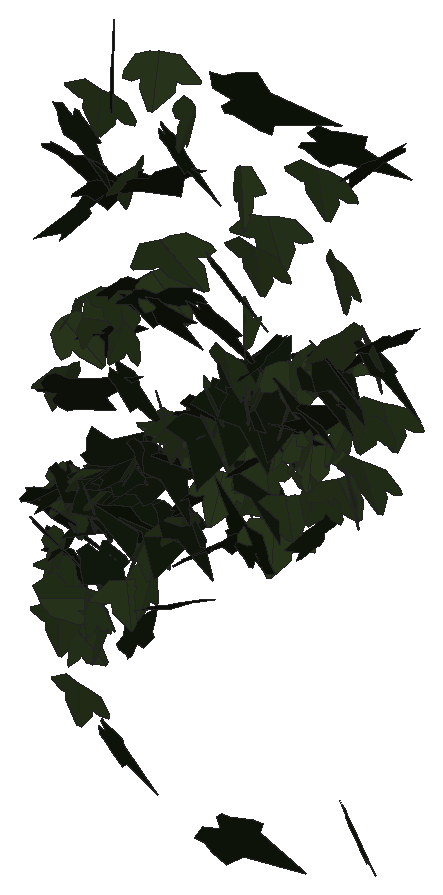
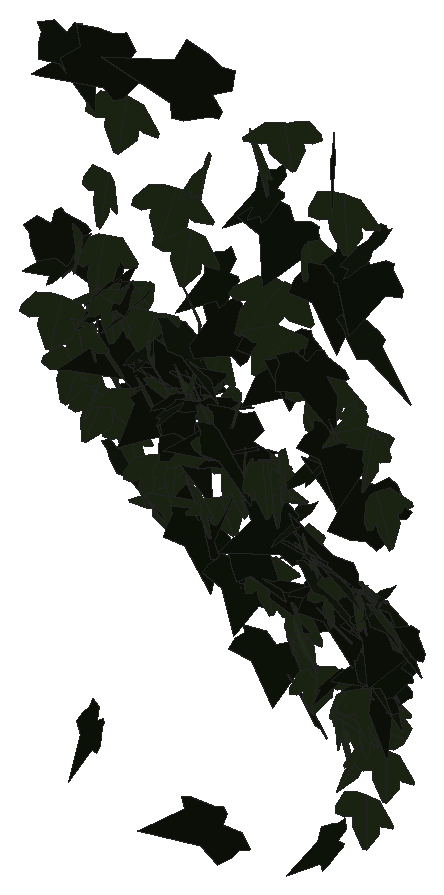
# SketchUp Ruby script. Lengths in inches.
U = 1.inch
M = Sketchup.active_model
def pt(a) = Geom::Point3d.new(a.map { |v| v * U })
def face(e, loops, mat)
  f = e.add_face(loops[0].map { |a| pt(a) })
  loops[1..].each { |l| e.add_face(l.map { |a| pt(a) }).erase! }
  f.material = f.back_material = mat if mat
  f
end
# faces: each face lists its corners as indices into pts; further lists are holes
def faces(e, pts, list, mat = nil) = list.each { |f| face(e, (f[0].is_a?(Array) ? f : [f]).map { |l| l.map { |i| pts[i] } }, mat) }
# xy, xz, yz: faces in a plane at the given z, y or x. An outline is a flat list of corners, or four numbers for a rectangle; further outlines are holes
def ring(l) = l.size == 4 ? [[l[0], l[1]], [l[2], l[1]], [l[2], l[3]], [l[0], l[3]]] : l.each_slice(2).to_a
def flat(e, list, mat, &to3) = list.each { |f| face(e, (f[0].is_a?(Array) ? f : [f]).map { |l| ring(l).map { |u, v| to3.(u, v) } }, mat) }
def xy(e, z, list, mat = nil) = flat(e, list, mat) { |x, y| [x, y, z] }
def xz(e, y, list, mat = nil) = flat(e, list, mat) { |x, z| [x, y, z] }
def yz(e, x, list, mat = nil) = flat(e, list, mat) { |y, z| [x, y, z] }
def lines(e, pts, list) = list.each { |a, b| e.add_line(pt(pts[a]), pt(pts[b])) }
# prism: a flat outline (further loops are holes) pulled along v
def prism(e, loops, v, mat = nil)
  f = face(e, loops, mat); d = Geom::Vector3d.new(v.map { |x| x * U })
  f.pushpull(f.normal.samedirection?(d) ? d.length : -d.length)
end
def box(e, o, s, mat = nil) = prism(e, [[o, [o[0] + s[0], o[1], o[2]], [o[0] + s[0], o[1] + s[1], o[2]], [o[0], o[1] + s[1], o[2]]]], [0, 0, s[2]], mat)
def at(x, y, z, deg = 0) = Geom::Transformation.translation(pt([x, y, z])) * Geom::Transformation.rotation(ORIGIN, Z_AXIS, deg.degrees)
def axes(o, x, y, z) = Geom::Transformation.new([*x, 0, *y, 0, *z, 0, *pt(o).to_a, 1])
def part(name) = M.definitions.add(name)
# library, detail: a bought-in or finely detailed component or shape, given as its bounding box
def library(name, o, s) = part(name).tap { |d| box(d.entities, o, s) }
def detail(e, o, s) = box(e.add_group.entities, o, s)
def put(e, d, t, mat = nil) = e.add_instance(d, t).tap { |i| i.material = mat if mat }
def group(e, t, mat = nil) = e.add_group.tap { |g| g.transformation = t; g.material = mat if mat }.entities
root = M.entities
M.materials.add("1026 AP 7946 SUNNY SIDE UP").color = [254, 231, 186]
M.materials.add("efeu1").color = [18, 25, 13]
M.materials.add("efeu2").color = [43, 57, 29]
c1 = part("ivyleaf_9")
p = [[1.54,2.16,1.25],[1.36,2.04,1.19],[-0.21,0.99,0.68],[-0.71,1.11,0.82],[-0.85,0.86,0.67],[-0.8,0.17,0.21],
  [-0.9,-0.01,0.1],[-0.67,-0.16,-0.02],[-0.08,-0.08,-0.05],[-0.03,-0.6,-0.4],[0.65,-0.88,-0.66],[0.83,-0.6,-0.49],
  [1.29,-0.42,-0.43],[1.8125,-0.07,-0.26],[1.21,0.44,0.15]]
faces(c1.entities,p,[[0,1,2,3,4,5,6,7,8,9,10,11,12,13,14]],"efeu1")
c2 = part("ivyleaf_10")
p = [[0,0.5,-0.03],[-0.0625,2.02,-0.43],[-0.19,2.01,-0.46],[-0.54,1.05,-0.29],[-0.52,0.625,-0.18],[-0.83,0.76,-0.28],
  [-1.16,0.64,-0.33],[-1.15,0.33,-0.24],[-0.77,-0.39,0.02],[-0.3,-0.51,0.16],[0.04,-0.48,0.23],[-0.02,2.01,-0.4375],
  [-0.06,2.01,-0.43],[0.04,-0.49,0.23],[0.67,-0.49,0.14],[1.38,0.36,-0.2],[1.375,0.51,-0.24],[0.81,0.65,-0.19],
  [0.62,0.59,-0.15],[0.6,1.09,-0.28],[0.5,1.23,-0.31]]
faces(c2.entities,p,[[0,1,2,3,4,5,6,7,8,9,10],[11,12,0,13,14,15,16,17,18,19,20]],"efeu2")
put(root,c1,axes([122.53,212.98,271.5625],[0.22662,-0.02057,-0.23911],[-0.36508,0.00859,-0.14934],[0.02856,0.27297,-0.01171]),"1026 AP 7946 SUNNY SIDE UP")
put(root,c2,axes([122.51,212.89,270.52],[-0.4181,0.04854,0.03929],[-0.06821,-0.02864,-0.27619],[-0.06868,-0.26705,0.03513]),"1026 AP 7946 SUNNY SIDE UP")
put(root,c1,axes([122.42,212.8125,272.46],[0.27398,0.21836,-0.00939],[0.003,-0.01477,-0.28767],[-0.34373,0.17392,-0.01]),"1026 AP 7946 SUNNY SIDE UP")
put(root,c1,axes([122.69,212.7,272.61],[-0.18146,0.2621,0.02234],[-0.03851,0.01125,-0.29439],[-0.41154,-0.11662,0.01769]),"1026 AP 7946 SUNNY SIDE UP")
put(root,c2,axes([122.48,212.86,271.68],[0.2605,-0.21806,0.00555],[0.00539,-0.00571,-0.28216],[0.343,0.1657,0.00022]),"1026 AP 7946 SUNNY SIDE UP")
put(root,c1,axes([122.22,212.87,271.77],[0.34565,-0.16054,0.06421],[0.08155,-0.03622,-0.28063],[0.25877,0.22585,0.00267]),"1026 AP 7946 SUNNY SIDE UP")
put(root,c1,axes([122.22,212.97,272.04],[0.39548,-0.09969,0.06037],[0.0993,-0.0007,-0.27779],[0.15286,0.25838,0.02427]),"1026 AP 7946 SUNNY SIDE UP")
put(root,c1,axes([122.72,212.87,271.83],[-0.14965,0.25687,0.02102],[-0.01059,0.01771,-0.2821],[-0.40485,-0.09541,-0.00039]),"1026 AP 7946 SUNNY SIDE UP")
put(root,c2,axes([122.61,212.83,274.26],[-0.0857,-0.28398,0.0248],[0.00631,-0.02691,-0.29791],[0.44831,-0.05391,0.00894]),"1026 AP 7946 SUNNY SIDE UP")
put(root,c2,axes([122.68,212.96,271.38],[-0.35392,-0.15518,0.00923],[0.01173,-0.02808,-0.2804],[0.24422,-0.22354,0.02685]),"1026 AP 7946 SUNNY SIDE UP")
put(root,c2,axes([122.67,212.89,272.67],[0.34306,-0.17608,-0.00482],[-0.02989,-0.01772,-0.28772],[0.27531,0.21749,-0.02523]),"1026 AP 7946 SUNNY SIDE UP")
put(root,c1,axes([122.95,212.88,276.79],[-0.28904,0.26922,-0.05345],[0.02471,-0.05386,-0.33568],[-0.43086,-0.18369,0.01661]),"1026 AP 7946 SUNNY SIDE UP")
put(root,c2,axes([122.73,212.84,272.46],[-0.43019,0.06143,-0.01948],[0.01444,-0.04598,-0.28576],[-0.10019,-0.27038,0.04246]),"1026 AP 7946 SUNNY SIDE UP")
put(root,c2,axes([122.72,212.84,275.11],[0.01575,-0.25454,-0.15111],[0.06267,0.14515,-0.2584],[0.45653,-0.01114,0.04069]),"1026 AP 7946 SUNNY SIDE UP")
put(root,c2,axes([122.49,212.77,270.88],[-0.12444,-0.04589,0.27298],[0.31916,0.17142,0.09395],[-0.27802,0.21733,-0.01434]),"1026 AP 7946 SUNNY SIDE UP")
put(root,c2,axes([122.84,212.89,272.71],[0.02726,-0.28212,0.00318],[-0.00747,-0.00499,-0.29117],[0.4436,0.01725,-0.0051]),"1026 AP 7946 SUNNY SIDE UP")
put(root,c2,axes([122.93,212.78,269.65],[-0.41498,0.05647,0.05341],[-0.08683,-0.01276,-0.27705],[-0.08312,-0.2686,0.02274]),"1026 AP 7946 SUNNY SIDE UP")
put(root,c1,axes([122.67,212.86,272.75],[0.22083,-0.23889,-0.06244],[-0.02541,0.05912,-0.28468],[0.38618,0.1405,0.01697]),"1026 AP 7946 SUNNY SIDE UP")
put(root,c1,axes([122.91,212.72,277.63],[0.39161,0.12084,-0.14425],[-0.24313,0.00515,-0.27735],[-0.16108,0.28601,0.06792]),"1026 AP 7946 SUNNY SIDE UP")
put(root,c2,axes([123,212.89,270.93],[-0.37994,0.12302,0.04689],[-0.12258,-0.0596,-0.26481],[-0.1654,-0.23842,0.08853]),"1026 AP 7946 SUNNY SIDE UP")
put(root,c1,axes([122.7,212.93,278.03],[0.19808,-0.2736,0.03914],[0.0193,-0.03788,-0.31049],[0.43425,0.12648,-0.00405]),"1026 AP 7946 SUNNY SIDE UP")
put(root,c1,axes([122.64,212.73,274.01],[0.37365,0.20279,-0.10254],[0.0843,0.09141,0.32056],[0.34589,-0.24135,0.03264]),"1026 AP 7946 SUNNY SIDE UP")
put(root,c2,axes([122.96,212.8,272.7],[-0.23019,0.23958,-0.02362],[-0.00051,-0.02862,-0.28899],[-0.37865,-0.14561,0.01475]),"1026 AP 7946 SUNNY SIDE UP")
put(root,c2,axes([122.86,212.68,275.07],[0.16423,0.22664,0.16237],[0.09304,0.14481,-0.25617],[-0.42281,0.1199,0.0067]),"1026 AP 7946 SUNNY SIDE UP")
put(root,c2,axes([122.93,212.82,270.44],[-0.01642,-0.23407,-0.1501],[0.16525,0.13011,-0.2244],[0.39961,-0.06343,0.08663]),"1026 AP 7946 SUNNY SIDE UP")
put(root,c1,axes([123.12,212.94,272.7],[0.25806,0.17161,-0.15313],[-0.14303,-0.11965,-0.24488],[-0.32818,0.18709,-0.01369]),"1026 AP 7946 SUNNY SIDE UP")
put(root,c2,axes([123.18,212.92,278.52],[-0.471,0.01526,0.05824],[-0.09073,-0.02956,-0.30741],[-0.01485,-0.30338,0.03108]),"1026 AP 7946 SUNNY SIDE UP")
put(root,c1,axes([123.16,212.91,275.02],[0.15872,0.2741,-0.01722],[0.0043,-0.02047,-0.30087],[-0.43193,0.10052,-0.00932]),"1026 AP 7946 SUNNY SIDE UP")
put(root,c2,axes([123.24,212.85,271.09],[-0.22518,0.18129,0.15871],[-0.1698,0.10934,-0.23692],[-0.33215,-0.1788,0.01353]),"1026 AP 7946 SUNNY SIDE UP")
put(root,c1,axes([123.35,213.01,272.41],[-0.38475,0.12561,-0.03026],[0.02544,-0.03414,-0.28257],[-0.2015,-0.24416,0.02211]),"1026 AP 7946 SUNNY SIDE UP")
put(root,c2,axes([123.17,212.95,272.86],[-0.31044,-0.18987,-0.04619],[0.08707,0.00506,-0.27994],[0.29375,-0.20216,0.03416]),"1026 AP 7946 SUNNY SIDE UP")
put(root,c2,axes([123.13,212.69,275.34],[0.0015,-0.14596,-0.26552],[0.15493,0.24236,-0.14006],[0.43801,-0.08523,0.05045]),"1026 AP 7946 SUNNY SIDE UP")
put(root,c2,axes([123.29,212.77,270.61],[0.16619,-0.24356,-0.07999],[-0.0398,0.07213,-0.27304],[0.39933,0.10855,0.00608]),"1026 AP 7946 SUNNY SIDE UP")
put(root,c2,axes([123.27,212.93,272.65],[0.00886,-0.27426,0.05014],[0.02142,-0.04991,-0.2826],[0.43789,0.00799,0.01281]),"1026 AP 7946 SUNNY SIDE UP")
put(root,c1,axes([123.11,212.96,271.67],[0.11195,-0.23955,-0.11981],[-0.05845,0.10884,-0.25678],[0.41367,0.08021,-0.00386]),"1026 AP 7946 SUNNY SIDE UP")
put(root,c1,axes([123.33,212.89,277.34],[0.13376,0.28654,-0.04761],[-0.01271,-0.0475,-0.30815],[-0.45662,0.08526,-0.00537]),"1026 AP 7946 SUNNY SIDE UP")
put(root,c1,axes([123.57,212.96,272.94],[-0.22552,0.2392,0.02733],[-0.04485,0.01219,-0.28665],[-0.37553,-0.1451,0.01782]),"1026 AP 7946 SUNNY SIDE UP")
put(root,c1,axes([123.47,212.74,278.71],[0.01476,-0.09243,0.32751],[0.08567,0.31467,0.09428],[-0.5143,0.04976,0.0251]),"1026 AP 7946 SUNNY SIDE UP")
put(root,c2,axes([123.58,212.88,275.2],[-0.34307,0.17362,0.10312],[-0.21622,-0.02384,-0.26896],[-0.22818,-0.23845,0.09983]),"1026 AP 7946 SUNNY SIDE UP")
put(root,c1,axes([123.72,212.9,273.18],[-0.35005,0.16297,0.04746],[-0.11718,-0.02755,-0.27629],[-0.23869,-0.22548,0.06603]),"1026 AP 7946 SUNNY SIDE UP")
put(root,c1,axes([123.68,212.82,273.24],[-0.18259,0.24752,0.06637],[-0.09761,0.0398,-0.27865],[-0.38958,-0.12598,0.03871]),"1026 AP 7946 SUNNY SIDE UP")
put(root,c1,axes([123.28,212.93,269.0625],[0.32843,-0.17099,-0.07704],[-0.07189,0.06044,-0.27717],[0.28389,0.21313,0.01894]),"1026 AP 7946 SUNNY SIDE UP")
put(root,c1,axes([123.31,212.93,273.03],[-0.2044,0.12307,0.22651],[0.26161,-0.14283,0.18345],[0.29627,0.21103,-0.00571]),"1026 AP 7946 SUNNY SIDE UP")
put(root,c2,axes([123.54,212.87,275.68],[-0.41037,-0.1408,-0.00756],[0.02713,-0.01825,-0.30458],[0.21996,-0.26043,0.02346]),"1026 AP 7946 SUNNY SIDE UP")
put(root,c1,axes([123.39,212.875,272.74],[-0.13371,-0.23152,-0.14557],[0.08717,0.12872,-0.25325],[0.4164,-0.10129,0.00627]),"1026 AP 7946 SUNNY SIDE UP")
put(root,c1,axes([123.73,212.92,275.98],[0.01893,0.26471,-0.1366],[-0.00313,-0.13414,-0.27375],[-0.46659,0.01164,-0.0037]),"1026 AP 7946 SUNNY SIDE UP")
put(root,c2,axes([123.61,212.89,271.37],[-0.23173,-0.2347,-0.00504],[0.11421,-0.04161,-0.27243],[0.35096,-0.14142,0.08533]),"1026 AP 7946 SUNNY SIDE UP")
put(root,c2,axes([123.69,212.89,277.6],[0.00022,-0.30207,-0.03698],[0.02241,0.03415,-0.31065],[0.47748,-0.00147,0.0146]),"1026 AP 7946 SUNNY SIDE UP")
put(root,c1,axes([123.96,212.97,273.1875],[-0.41614,0.06145,0.06559],[-0.11207,-0.03085,-0.27622],[-0.0818,-0.27037,0.04474]),"1026 AP 7946 SUNNY SIDE UP")
put(root,c2,axes([123.73,212.91,273.35],[0.12216,-0.27441,-0.00467],[-0.00148,0.00283,-0.29379],[0.43151,0.0777,0.00032]),"1026 AP 7946 SUNNY SIDE UP")
put(root,c2,axes([123.77,213.04,272.1],[0.13573,-0.26106,0.02199],[-0.00235,-0.02453,-0.28325],[0.41205,0.08586,-0.00886]),"1026 AP 7946 SUNNY SIDE UP")
put(root,c1,axes([123.92,212.71,270.78],[0.02853,0.1117,0.26242],[-0.08119,0.25155,-0.10865],[-0.42882,-0.0402,0.03803]),"1026 AP 7946 SUNNY SIDE UP")
put(root,c1,axes([123.59,212.8,274.57],[0.31078,-0.1877,-0.10864],[-0.08245,0.09541,-0.27843],[0.3275,0.20214,0.033]),"1026 AP 7946 SUNNY SIDE UP")
put(root,c1,axes([123.5,212.8125,272.35],[0.22303,-0.05599,0.23681],[0.34559,-0.06904,-0.15722],[0.13903,0.26142,0.01091]),"1026 AP 7946 SUNNY SIDE UP")
put(root,c2,axes([123.96,212.87,271.65],[0.32907,-0.18368,0.02519],[0.04112,-0.00883,-0.2867],[0.28867,0.21064,0.01212]),"1026 AP 7946 SUNNY SIDE UP")
put(root,c2,axes([123.93,212.9,272.16],[0.3955,-0.11882,0.03464],[0.08854,0.04083,-0.27948],[0.17313,0.25055,0.0638]),"1026 AP 7946 SUNNY SIDE UP")
put(root,c2,axes([124.09,212.94,279.33],[0.33872,0.21842,-0.03574],[-0.06636,-0.00869,-0.31514],[-0.34168,0.21822,0.02578]),"1026 AP 7946 SUNNY SIDE UP")
put(root,c1,axes([123.94,212.9,273.56],[0.24274,-0.23659,-0.04875],[0.00307,0.05583,-0.28887],[0.37897,0.15109,0.03356]),"1026 AP 7946 SUNNY SIDE UP")
put(root,c1,axes([124.01,212.76,275.82],[0.46248,0.04372,-0.00493],[-0.00837,0.00163,-0.30631],[-0.06869,0.29416,0.00418]),"1026 AP 7946 SUNNY SIDE UP")
put(root,c1,axes([124.28,212.69,276.08],[0.19879,0.25686,-0.09471],[-0.06036,-0.08519,-0.29541],[-0.42549,0.13209,-0.00234]),"1026 AP 7946 SUNNY SIDE UP")
put(root,c2,axes([124.31,212.74,274.22],[0.11696,-0.13389,-0.2521],[-0.0805,0.24162,-0.15128],[0.43009,0.08163,0.04024]),"1026 AP 7946 SUNNY SIDE UP")
put(root,c1,axes([124.2,212.67,277.79],[0.24345,0.26572,0.05119],[0.03819,0.04162,-0.31658],[-0.42291,0.15672,0.00088]),"1026 AP 7946 SUNNY SIDE UP")
put(root,c1,axes([124.24,213.01,272.6],[-0.31463,-0.18184,-0.07247],[0.12961,0.01086,-0.27443],[0.27718,-0.21148,0.04607]),"1026 AP 7946 SUNNY SIDE UP")
put(root,c1,axes([124.05,212.91,273.41],[0.35077,0.09967,0.14115],[0.17449,0.084,-0.24962],[-0.20036,0.24764,0.02972]),"1026 AP 7946 SUNNY SIDE UP")
put(root,c1,axes([124.42,212.76,271.48],[0.16466,0.25888,0.01615],[-0.09402,0.03903,-0.27828],[-0.39668,0.09821,0.07266]),"1026 AP 7946 SUNNY SIDE UP")
put(root,c1,axes([124.18,212.98,273.5],[0.0895,-0.27643,-0.00918],[-0.00391,0.00698,-0.29071],[0.4348,0.05697,-0.00073]),"1026 AP 7946 SUNNY SIDE UP")
put(root,c2,axes([124.21,212.83,276.15],[0.23369,0.21091,0.15598],[0.09697,0.13938,-0.26365],[-0.39543,0.15882,0.02752]),"1026 AP 7946 SUNNY SIDE UP")
put(root,c2,axes([124.39,212.87,274.04],[0.31435,-0.18421,-0.10323],[-0.03272,0.11897,-0.2702],[0.32731,0.1888,0.07213]),"1026 AP 7946 SUNNY SIDE UP")
put(root,c2,axes([124.43,212.96,274.15],[-0.16461,-0.26685,-0.02071],[0.02313,0.01419,-0.29509],[0.41998,-0.10537,0.00813]),"1026 AP 7946 SUNNY SIDE UP")
put(root,c2,axes([124.71,212.9,273.98],[0.09063,-0.02861,-0.28955],[-0.43412,0.05435,-0.06374],[0.093,0.28156,-0.01539]),"1026 AP 7946 SUNNY SIDE UP")
put(root,c2,axes([124.48,212.9,272.65],[-0.14711,-0.266,0.00922],[0.00787,-0.01285,-0.29042],[0.41851,-0.09326,0.00871]),"1026 AP 7946 SUNNY SIDE UP")
put(root,c2,axes([124.38,212.8,276.75],[-0.37433,-0.18716,-0.1729],[0.24526,0.06946,-0.30927],[0.30858,-0.28225,0.03607]),"1026 AP 7946 SUNNY SIDE UP")
put(root,c2,axes([124.56,212.88,274.12],[-0.0632,-0.28561,0.02529],[0.00224,-0.02662,-0.29724],[0.45097,-0.03989,0.00502]),"1026 AP 7946 SUNNY SIDE UP")
put(root,c1,axes([124.62,213.1,273.07],[-0.14296,0.19611,-0.18246],[0.10377,-0.16573,-0.22352],[-0.40355,-0.11209,0.00716]),"1026 AP 7946 SUNNY SIDE UP")
put(root,c1,axes([124.34,212.86,278.33],[0.36262,-0.18799,-0.07964],[-0.08484,0.05443,-0.30609],[0.30749,0.23671,0.00946]),"1026 AP 7946 SUNNY SIDE UP")
put(root,c1,axes([124.39,212.96,272.74],[0.14282,-0.25807,-0.06234],[-0.00789,0.06074,-0.28107],[0.41621,0.08971,0.01607]),"1026 AP 7946 SUNNY SIDE UP")
put(root,c2,axes([124.67,212.83,278.82],[0.28075,-0.25454,-0.02477],[0.00565,0.03007,-0.31945],[0.40177,0.17745,0.0218]),"1026 AP 7946 SUNNY SIDE UP")
put(root,c1,axes([124.88,212.85,272.39],[0.10384,0.26336,0.08493],[-0.0028,0.08365,-0.27837],[-0.43322,0.06258,0.02216]),"1026 AP 7946 SUNNY SIDE UP")
put(root,c2,axes([124.89,212.97,274],[-0.07039,-0.28131,0.00393],[0.00132,-0.00561,-0.29348],[0.44242,-0.04474,0.0015]),"1026 AP 7946 SUNNY SIDE UP")
put(root,c1,axes([125.125,212.98,274.46],[-0.10653,0.27541,-0.02646],[-0.00176,-0.02832,-0.29224],[-0.43516,-0.06731,0.00766]),"1026 AP 7946 SUNNY SIDE UP")
put(root,c1,axes([125,212.97,274.19],[-0.20783,-0.25012,0.01763],[0.002,-0.02162,-0.29134],[0.39437,-0.13171,0.01076]),"1026 AP 7946 SUNNY SIDE UP")
put(root,c1,axes([124.77,212.85,274.45],[0.35382,0.06499,0.18281],[0.27268,0.03719,-0.24086],[-0.11671,0.28392,-0.00852]),"1026 AP 7946 SUNNY SIDE UP")
put(root,c2,axes([125.12,212.73,274.85],[-0.25989,0.23751,0.03166],[-0.03534,0.02014,-0.29789],[-0.37465,-0.16666,0.00614]),"1026 AP 7946 SUNNY SIDE UP")
put(root,c2,axes([125.06,212.84,274.29],[-0.34345,0.16434,-0.09913],[0.10394,-0.0734,-0.28143],[-0.28163,-0.22751,0.01703]),"1026 AP 7946 SUNNY SIDE UP")
put(root,c2,axes([125.13,212.95,273.45],[0.28767,0.20395,-0.07156],[-0.07182,-0.05389,-0.28256],[-0.33169,0.18855,-0.00088]),"1026 AP 7946 SUNNY SIDE UP")
put(root,c1,axes([125,212.77,276.02],[0.45615,-0.07835,0.00611],[-0.00189,-0.02882,-0.30837],[0.12358,0.28873,-0.02729]),"1026 AP 7946 SUNNY SIDE UP")
put(root,c2,axes([125.2,212.97,274.31],[-0.00103,-0.28061,0.05616],[-0.00105,0.05611,0.28941],[-0.44996,0.00051,-0.00081]),"1026 AP 7946 SUNNY SIDE UP")
put(root,c2,axes([125.42,212.77,275.4375],[-0.41318,0.14647,0.00058],[-0.02317,-0.02699,-0.30845],[-0.22914,-0.26138,0.03015]),"1026 AP 7946 SUNNY SIDE UP")
put(root,c1,axes([125.2,212.78,276.75],[0.39129,-0.15497,-0.07044],[-0.09079,0.03497,-0.3018],[0.2498,0.25546,0.00065]),"1026 AP 7946 SUNNY SIDE UP")
put(root,c1,axes([125.6,212.85,272.93],[0.03028,0.28375,-0.02797],[0.00023,-0.02884,-0.29315],[-0.44846,0.01915,-0.00204]),"1026 AP 7946 SUNNY SIDE UP")
put(root,c2,axes([125.53,213.04,273.5],[0.28375,-0.21296,-0.04515],[-0.03956,0.03453,-0.28734],[0.3392,0.18218,0.00425]),"1026 AP 7946 SUNNY SIDE UP")
put(root,c1,axes([125.5,212.94,274.8],[-0.254,-0.23795,-0.03618],[0.0545,0.0172,-0.29555],[0.37396,-0.16413,0.0185]),"1026 AP 7946 SUNNY SIDE UP")
put(root,c2,axes([125.55,212.97,274.12],[0.16927,0.24316,-0.1028],[-0.07392,-0.0898,-0.2744],[-0.40747,0.1173,0.00708]),"1026 AP 7946 SUNNY SIDE UP")
put(root,c2,axes([125.72,212.76,275.85],[0.19667,-0.09682,0.26407],[-0.28258,0.18451,0.16286],[-0.3263,-0.21814,0.01812]),"1026 AP 7946 SUNNY SIDE UP")
put(root,c1,axes([125.8125,212.75,272.71],[0.11795,-0.1528,0.30685],[-0.18417,0.27492,0.17678],[-0.49441,-0.13886,0.00735]),"1026 AP 7946 SUNNY SIDE UP")
put(root,c2,axes([125.58,212.85,278.17],[-0.01256,0.28586,-0.11493],[-0.00635,-0.11331,-0.29519],[-0.4834,-0.00594,0.00686]),"1026 AP 7946 SUNNY SIDE UP")
put(root,c2,axes([125.69,212.78,275.19],[-0.14543,0.27511,-0.03137],[-0.05019,-0.04412,-0.2958],[-0.4326,-0.08737,0.04486]),"1026 AP 7946 SUNNY SIDE UP")
put(root,c1,axes([125.375,212.71,268.47],[0.05367,0.01583,-0.29584],[0.28675,0.22254,0.03626],[0.34988,-0.18482,0.01566]),"1026 AP 7946 SUNNY SIDE UP")
put(root,c2,axes([125.77,212.9,277.09],[-0.46585,0.05674,0.02308],[-0.04033,-0.01681,-0.31008],[-0.08683,-0.29661,0.02018]),"1026 AP 7946 SUNNY SIDE UP")
put(root,c1,axes([125.93,212.84,275.66],[-0.18156,0.27424,0.00294],[-0.01127,-0.00161,-0.30646],[-0.43107,-0.11546,0.00677]),"1026 AP 7946 SUNNY SIDE UP")
put(root,c1,axes([125.86,212.82,274.13],[-0.05141,0.26757,-0.09282],[0.02446,-0.09038,-0.2782],[-0.44404,-0.03596,-0.00458]),"1026 AP 7946 SUNNY SIDE UP")
put(root,c1,axes([125.72,212.92,275.03],[-0.32795,0.0477,0.20439],[0.31432,-0.00726,0.21854],[0.06234,0.28758,-0.02665]),"1026 AP 7946 SUNNY SIDE UP")
put(root,c2,axes([125.8,212.875,275.2],[0.2334,-0.2461,0.05083],[0.02272,-0.05047,-0.29604],[0.39445,0.14852,-0.01303]),"1026 AP 7946 SUNNY SIDE UP")
put(root,c1,axes([125.72,212.94,274.85],[-0.06588,-0.28115,-0.05952],[0.00832,0.05601,-0.29249],[0.45074,-0.04213,-0.0033]),"1026 AP 7946 SUNNY SIDE UP")
put(root,c2,axes([125.88,212.88,275.21],[0.13018,-0.27895,0.04231],[0.01002,-0.04259,-0.29995],[0.44361,0.08282,-0.00564]),"1026 AP 7946 SUNNY SIDE UP")
put(root,c1,axes([125.7,212.95,273.78],[0.0937,-0.27837,-0.00072],[-0.0023,-0.00121,-0.29327],[0.4377,0.05959,-0.00139]),"1026 AP 7946 SUNNY SIDE UP")
put(root,c2,axes([125.84,212.98,273.89],[-0.17863,-0.26144,-0.01151],[0.12366,-0.02405,-0.2815],[0.39235,-0.11145,0.08348]),"1026 AP 7946 SUNNY SIDE UP")
put(root,c1,axes([125.5,212.81,279.35],[0.26455,-0.01093,0.31728],[0.46721,-0.08759,-0.1709],[0.12891,0.33989,-0.03172]),"1026 AP 7946 SUNNY SIDE UP")
put(root,c1,axes([125.78,212.99,274.77],[0.21013,-0.25472,-0.00766],[0.00136,0.00721,-0.29626],[0.40063,0.13357,0.00502]),"1026 AP 7946 SUNNY SIDE UP")
put(root,c2,axes([126.02,212.89,277.62],[-0.42571,-0.13044,-0.0478],[0.09935,-0.0275,-0.30516],[0.19327,-0.27318,0.05157]),"1026 AP 7946 SUNNY SIDE UP")
put(root,c1,axes([126.08,212.98,275.0625],[-0.34015,-0.14617,-0.12808],[0.20556,0.02322,-0.26409],[0.21972,-0.24801,0.0488]),"1026 AP 7946 SUNNY SIDE UP")
put(root,c2,axes([126.05,212.87,273.09],[0.39907,0.1315,-0.00154],[0.01734,-0.02612,-0.29318],[-0.20608,0.25246,-0.02764]),"1026 AP 7946 SUNNY SIDE UP")
put(root,c2,axes([126.08,212.88,274.71],[0.44656,-0.01191,0.04046],[0.06091,-0.01436,-0.29263],[0.02162,0.28635,-0.01131]),"1026 AP 7946 SUNNY SIDE UP")
put(root,c1,axes([126.03,212.875,274.58],[0.42935,0.08806,0.00983],[0.01256,0.0047,-0.29553],[-0.13863,0.27316,0.00368]),"1026 AP 7946 SUNNY SIDE UP")
put(root,c2,axes([126.27,212.89,273.5625],[-0.3214,-0.1995,-0.02778],[0.08642,-0.01996,-0.28935],[0.30427,-0.20506,0.05284]),"1026 AP 7946 SUNNY SIDE UP")
put(root,c2,axes([126.23,212.99,275.16],[0.24874,-0.1855,0.15936],[0.13039,-0.1333,-0.25111],[0.35784,0.17752,-0.01928]),"1026 AP 7946 SUNNY SIDE UP")
put(root,c2,axes([126.43,212.77,275.625],[0.34919,0.18636,0.05142],[0.01958,0.06051,-0.29576],[-0.3023,0.21918,0.04024]),"1026 AP 7946 SUNNY SIDE UP")
put(root,c1,axes([126.33,212.86,275.36],[0.27893,-0.22614,-0.03185],[-0.01412,0.03058,-0.29567],[0.35835,0.17723,0.01314]),"1026 AP 7946 SUNNY SIDE UP")
put(root,c2,axes([126.61,212.83,274.66],[0.25362,-0.23936,-0.03995],[-0.03736,0.02911,-0.29716],[0.37911,0.163,-0.00256]),"1026 AP 7946 SUNNY SIDE UP")
put(root,c2,axes([126.84,212.84,273.96],[-0.40332,0.09589,0.10148],[-0.17466,-0.0236,-0.27597],[-0.12631,-0.27355,0.05757]),"1026 AP 7946 SUNNY SIDE UP")
put(root,c2,axes([126.65,212.96,274.52],[0.28495,0.21986,-0.04171],[-0.0547,-0.02538,-0.29347],[-0.34761,0.18422,0.01199]),"1026 AP 7946 SUNNY SIDE UP")
put(root,c2,axes([126.71,212.69,275.91],[0.06477,0.26852,0.12361],[-0.08135,0.12439,-0.27122],[-0.45425,0.01601,0.0662]),"1026 AP 7946 SUNNY SIDE UP")
put(root,c1,axes([126.98,212.73,273.44],[-0.22463,0.25106,0.00639],[-0.01843,-0.00117,-0.29738],[-0.39441,-0.14293,0.01026]),"1026 AP 7946 SUNNY SIDE UP")
put(root,c2,axes([126.87,212.85,278.66],[-0.48518,0.02602,0.00342],[-0.00896,-0.03001,-0.31764],[-0.04023,-0.30712,0.0295]),"1026 AP 7946 SUNNY SIDE UP")
put(root,c2,axes([126.95,212.96,275.88],[-0.18979,-0.26355,-0.03288],[0.03518,0.02319,-0.29829],[0.41567,-0.1223,0.01023]),"1026 AP 7946 SUNNY SIDE UP")
put(root,c1,axes([126.7,212.9,275.77],[0.1859,-0.2699,-0.02881],[0.00501,0.03022,-0.30299],[0.4264,0.11732,0.01612]),"1026 AP 7946 SUNNY SIDE UP")
put(root,c1,axes([126.66,212.77,275.03],[0.31676,0.10278,0.19161],[0.27095,0.06961,-0.23221],[-0.19418,0.26479,-0.01144]),"1026 AP 7946 SUNNY SIDE UP")
put(root,c2,axes([126.91,212.95,275.91],[0.27779,0.23114,-0.00242],[0.02352,-0.01603,-0.29897],[-0.36272,0.17598,-0.02124]),"1026 AP 7946 SUNNY SIDE UP")
put(root,c1,axes([126.97,212.8,276.02],[0.40615,-0.09879,-0.10116],[-0.15133,0.02135,-0.28442],[0.15748,0.27531,-0.01242]),"1026 AP 7946 SUNNY SIDE UP")
put(root,c1,axes([127.01,212.86,276.01],[0.14107,-0.24716,-0.1436],[-0.09208,0.12542,-0.26992],[0.43547,0.10659,-0.01055]),"1026 AP 7946 SUNNY SIDE UP")
put(root,c2,axes([127.2,212.83,277.41],[-0.3654,0.19466,0.01961],[-0.06232,-0.01964,-0.30961],[-0.30099,-0.23224,0.0403]),"1026 AP 7946 SUNNY SIDE UP")
put(root,c2,axes([127.17,212.92,275.02],[0.32826,-0.20037,0.02023],[0.00025,-0.02976,-0.29746],[0.31675,0.20767,-0.02073]),"1026 AP 7946 SUNNY SIDE UP")
put(root,c2,axes([127.24,212.77,276.41],[-0.15994,-0.28327,-0.11958],[0.07584,0.10424,-0.3093],[0.47438,-0.11217,0.00913]),"1026 AP 7946 SUNNY SIDE UP")
put(root,c2,axes([127.22,212.83,274.2],[-0.27872,-0.2119,-0.09802],[0.12607,0.05491,-0.28313],[0.34197,-0.19295,0.02449]),"1026 AP 7946 SUNNY SIDE UP")
put(root,c1,axes([126.97,212.75,279.24],[0.39839,0.05633,0.17563],[0.27215,-0.00027,-0.2654],[-0.07329,0.3052,-0.03081]),"1026 AP 7946 SUNNY SIDE UP")
put(root,c2,axes([127.49,213.04,275.2],[-0.43271,0.0507,0.08232],[-0.13418,-0.02873,-0.28517],[-0.06345,-0.28503,0.04165]),"1026 AP 7946 SUNNY SIDE UP")
put(root,c2,axes([127.36,212.84,274.31],[-0.18136,0.26458,-0.04562],[-0.00421,-0.05097,-0.29673],[-0.42219,-0.11315,0.02256]),"1026 AP 7946 SUNNY SIDE UP")
put(root,c1,axes([127.41,212.75,269.3],[0.32261,-0.12815,-0.17803],[-0.25366,0.06485,-0.24751],[0.22243,0.25981,-0.02405]),"1026 AP 7946 SUNNY SIDE UP")
put(root,c2,axes([127.64,212.83,274.57],[-0.45131,0.05176,-0.03495],[0.04619,-0.02929,-0.29965],[-0.08593,-0.28756,0.02248]),"1026 AP 7946 SUNNY SIDE UP")
put(root,c2,axes([127.625,212.9,276.42],[-0.26219,0.24203,-0.04572],[0.02121,-0.0462,-0.30266],[-0.38673,-0.16662,0.0144]),"1026 AP 7946 SUNNY SIDE UP")
put(root,c1,axes([127.88,212.72,279.32],[-0.05376,0.30402,-0.06748],[0.00945,-0.06697,-0.31556],[-0.48949,-0.03468,0.00132]),"1026 AP 7946 SUNNY SIDE UP")
put(root,c1,axes([127.93,212.96,276.58],[-0.11525,0.24042,-0.1593],[-0.00532,-0.16173,-0.2561],[-0.45061,-0.05958,0.04377]),"1026 AP 7946 SUNNY SIDE UP")
put(root,c2,axes([127.8125,213.01,275.4375],[-0.45039,-0.05295,-0.02097],[0.03813,-0.02125,-0.29908],[0.08045,-0.28635,0.02433]),"1026 AP 7946 SUNNY SIDE UP")
put(root,c1,axes([127.62,212.97,276.24],[0.26206,-0.24288,0.01281],[0.03011,-0.0036,-0.30315],[0.38134,0.16719,0.01513]),"1026 AP 7946 SUNNY SIDE UP")
